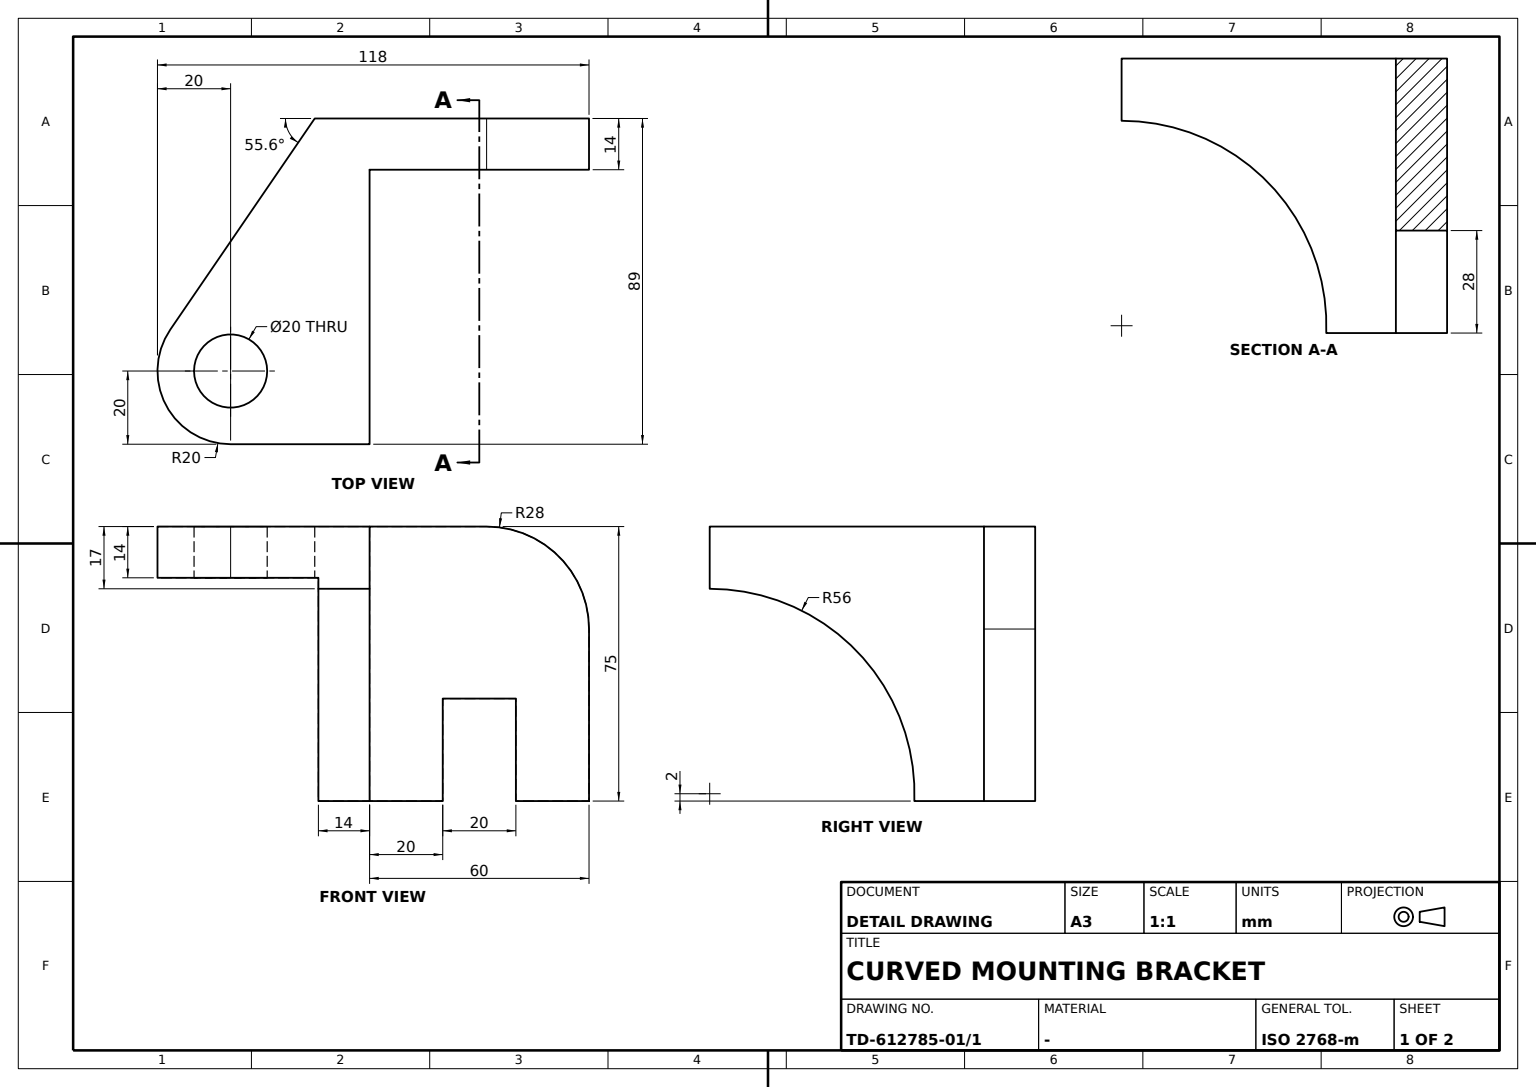
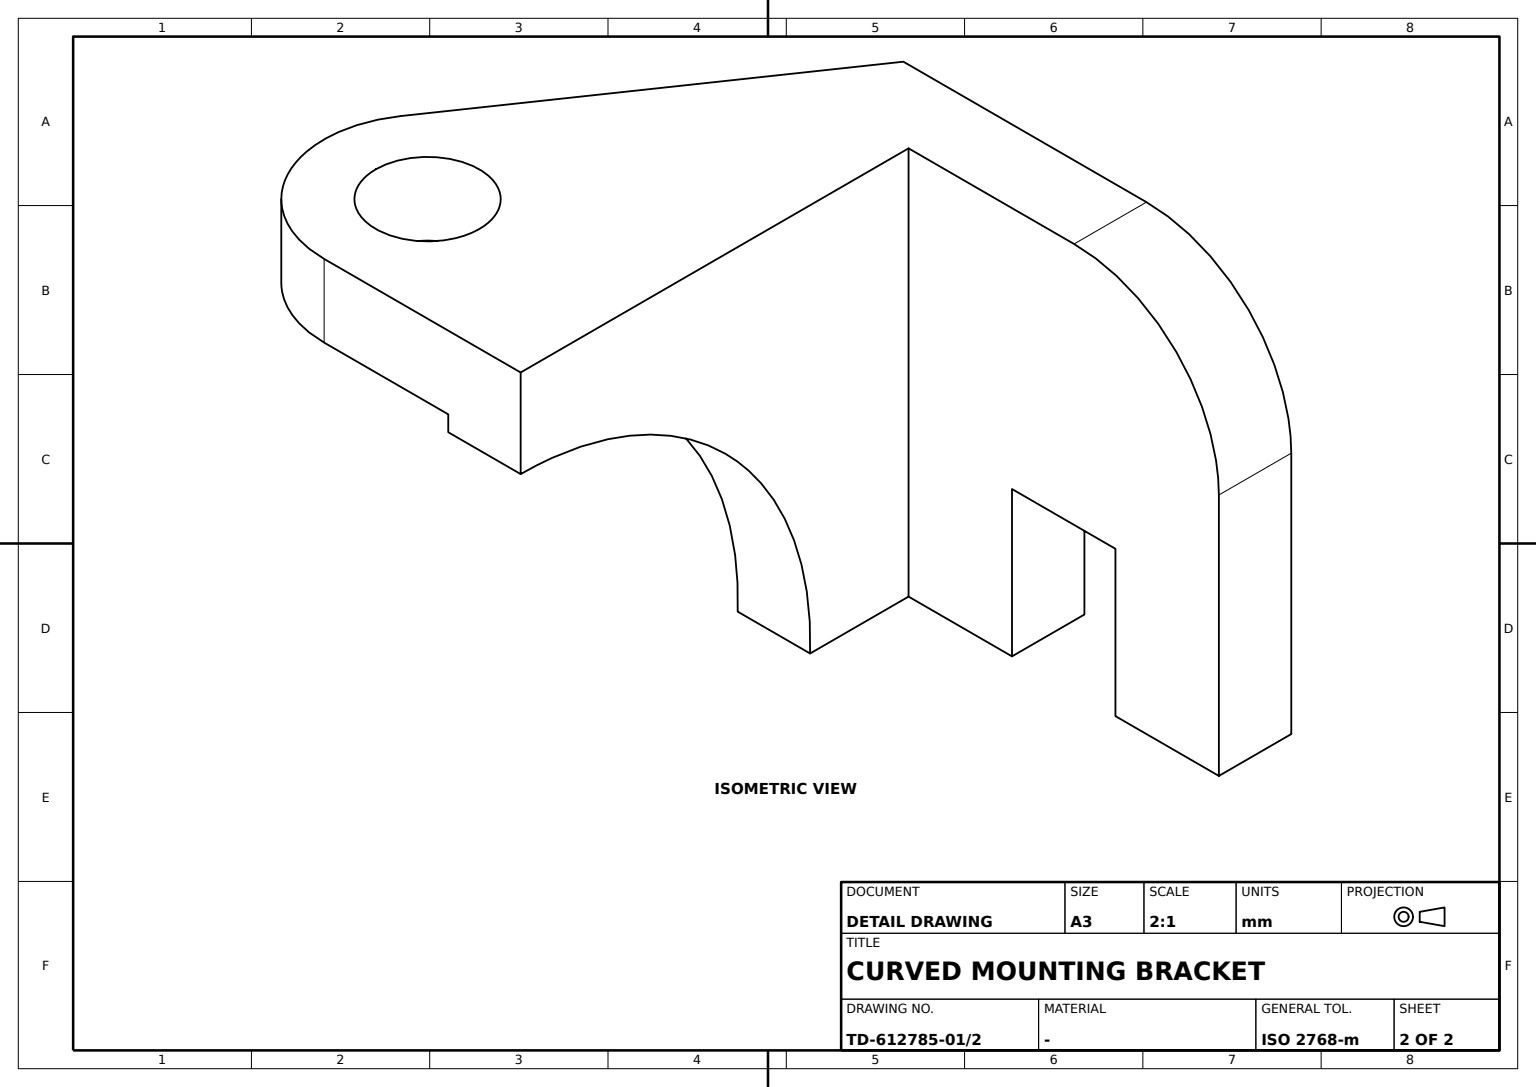
ISO-10303-21;
HEADER;
FILE_DESCRIPTION((''),'2;1');
FILE_NAME('','',(''),(''),'','','');
FILE_SCHEMA(('AUTOMOTIVE_DESIGN'));
ENDSEC;
DATA;
#1=APPLICATION_CONTEXT('');
#2=PRODUCT_CONTEXT('',#1,'mechanical');
#3=PRODUCT('','','',(#2));
#4=PRODUCT_DEFINITION_FORMATION('','',#3);
#5=PRODUCT_DEFINITION_CONTEXT('',#1,'design');
#6=PRODUCT_DEFINITION('','',#4,#5);
#7=PRODUCT_DEFINITION_SHAPE('','',#6);
#8=(LENGTH_UNIT()NAMED_UNIT(*)SI_UNIT(.MILLI.,.METRE.));
#9=(NAMED_UNIT(*)PLANE_ANGLE_UNIT()SI_UNIT($,.RADIAN.));
#10=(NAMED_UNIT(*)SI_UNIT($,.STERADIAN.)SOLID_ANGLE_UNIT());
#11=UNCERTAINTY_MEASURE_WITH_UNIT(LENGTH_MEASURE(0.005),#8,'distance_accuracy_value','');
#12=(GEOMETRIC_REPRESENTATION_CONTEXT(3)GLOBAL_UNCERTAINTY_ASSIGNED_CONTEXT((#11))GLOBAL_UNIT_ASSIGNED_CONTEXT((#8,#9,#10))REPRESENTATION_CONTEXT('',''));
#13=CARTESIAN_POINT('',(10.,0.,-37.5));
#14=VERTEX_POINT('',#13);
#15=CARTESIAN_POINT('',(10.,-14.,-37.5));
#16=VERTEX_POINT('',#15);
#17=CARTESIAN_POINT('',(10.,-29.,-37.5));
#18=DIRECTION('',(0.,1.,0.));
#19=VECTOR('',#18,1000.);
#20=LINE('',#17,#19);
#21=EDGE_CURVE('',#14,#16,#20,.F.);
#22=ORIENTED_EDGE('',*,*,#21,.T.);
#23=CARTESIAN_POINT('',(10.,-14.,-9.5));
#24=VERTEX_POINT('',#23);
#25=CARTESIAN_POINT('',(10.,-14.,0.));
#26=DIRECTION('',(0.,0.,-1.));
#27=VECTOR('',#26,1000.);
#28=LINE('',#25,#27);
#29=EDGE_CURVE('',#24,#16,#28,.T.);
#30=ORIENTED_EDGE('',*,*,#29,.F.);
#31=CARTESIAN_POINT('',(10.,0.,-9.5));
#32=VERTEX_POINT('',#31);
#33=CARTESIAN_POINT('',(10.,-29.,-9.5));
#34=LINE('',#33,#19);
#35=EDGE_CURVE('',#32,#24,#34,.F.);
#36=ORIENTED_EDGE('',*,*,#35,.F.);
#37=CARTESIAN_POINT('',(10.,0.,37.5));
#38=LINE('',#37,#27);
#39=EDGE_CURVE('',#32,#14,#38,.T.);
#40=ORIENTED_EDGE('',*,*,#39,.T.);
#41=EDGE_LOOP('',(#22,#30,#36,#40));
#42=FACE_BOUND('',#41,.T.);
#43=DIRECTION('',(1.,0.,0.));
#44=AXIS2_PLACEMENT_3D('',#33,#43,#26);
#45=PLANE('',#44);
#46=ADVANCED_FACE('',(#42),#45,.F.);
#47=CARTESIAN_POINT('',(-30.,-89.,20.5));
#48=VERTEX_POINT('',#47);
#49=CARTESIAN_POINT('',(-44.,-89.,20.5));
#50=VERTEX_POINT('',#49);
#51=DIRECTION('',(-1.,0.,0.));
#52=VECTOR('',#51,1000.);
#53=LINE('',#47,#52);
#54=EDGE_CURVE('',#48,#50,#53,.T.);
#55=ORIENTED_EDGE('',*,*,#54,.T.);
#56=CARTESIAN_POINT('',(-44.,-33.035726,-37.5));
#57=VERTEX_POINT('',#56);
#58=CARTESIAN_POINT('',(-44.,-89.,-35.5));
#59=DIRECTION('',(0.,0.,1.));
#60=AXIS2_PLACEMENT_3D('',#58,#51,#59);
#61=CIRCLE('',#60,56.);
#62=EDGE_CURVE('',#50,#57,#61,.T.);
#63=ORIENTED_EDGE('',*,*,#62,.T.);
#64=CARTESIAN_POINT('',(-30.,-33.035726,-37.5));
#65=VERTEX_POINT('',#64);
#66=CARTESIAN_POINT('',(-73.,-33.035726,-37.5));
#67=VECTOR('',#43,1000.);
#68=LINE('',#66,#67);
#69=EDGE_CURVE('',#57,#65,#68,.T.);
#70=ORIENTED_EDGE('',*,*,#69,.T.);
#71=CARTESIAN_POINT('',(-30.,-89.,-35.5));
#72=AXIS2_PLACEMENT_3D('',#71,#43,#18);
#73=CIRCLE('',#72,56.);
#74=EDGE_CURVE('',#65,#48,#73,.T.);
#75=ORIENTED_EDGE('',*,*,#74,.T.);
#76=EDGE_LOOP('',(#55,#63,#70,#75));
#77=FACE_BOUND('',#76,.T.);
#78=CARTESIAN_POINT('',(-73.,-89.,-35.5));
#79=AXIS2_PLACEMENT_3D('',#78,#43,#26);
#80=CYLINDRICAL_SURFACE('',#79,56.);
#81=ADVANCED_FACE('',(#77),#80,.F.);
#82=CARTESIAN_POINT('',(-68.,-89.,37.5));
#83=VERTEX_POINT('',#82);
#84=CARTESIAN_POINT('',(-84.503096,-57.701867,37.5));
#85=VERTEX_POINT('',#84);
#86=CARTESIAN_POINT('',(-68.,-69.,37.5));
#87=AXIS2_PLACEMENT_3D('',#86,#26,#43);
#88=CIRCLE('',#87,20.);
#89=EDGE_CURVE('',#83,#85,#88,.T.);
#90=ORIENTED_EDGE('',*,*,#89,.T.);
#91=CARTESIAN_POINT('',(-84.503096,-57.701867,23.5));
#92=VERTEX_POINT('',#91);
#93=LINE('',#84,#27);
#94=EDGE_CURVE('',#85,#92,#93,.T.);
#95=ORIENTED_EDGE('',*,*,#94,.T.);
#96=CARTESIAN_POINT('',(-68.,-89.,23.5));
#97=VERTEX_POINT('',#96);
#98=CARTESIAN_POINT('',(-68.,-69.,23.5));
#99=AXIS2_PLACEMENT_3D('',#98,#26,#43);
#100=CIRCLE('',#99,20.);
#101=EDGE_CURVE('',#97,#92,#100,.T.);
#102=ORIENTED_EDGE('',*,*,#101,.F.);
#103=LINE('',#82,#27);
#104=EDGE_CURVE('',#83,#97,#103,.T.);
#105=ORIENTED_EDGE('',*,*,#104,.F.);
#106=EDGE_LOOP('',(#90,#95,#102,#105));
#107=FACE_BOUND('',#106,.T.);
#108=AXIS2_PLACEMENT_3D('',#86,#26,#51);
#109=CYLINDRICAL_SURFACE('',#108,20.);
#110=ADVANCED_FACE('',(#107),#109,.T.);
#111=CARTESIAN_POINT('',(-30.,-89.,37.5));
#112=VERTEX_POINT('',#111);
#113=CARTESIAN_POINT('',(-44.,-89.,37.5));
#114=LINE('',#113,#67);
#115=EDGE_CURVE('',#112,#83,#114,.F.);
#116=ORIENTED_EDGE('',*,*,#115,.T.);
#117=ORIENTED_EDGE('',*,*,#104,.T.);
#118=CARTESIAN_POINT('',(-44.,-89.,23.5));
#119=VERTEX_POINT('',#118);
#120=CARTESIAN_POINT('',(-30.,-89.,23.5));
#121=LINE('',#120,#52);
#122=EDGE_CURVE('',#119,#97,#121,.T.);
#123=ORIENTED_EDGE('',*,*,#122,.F.);
#124=VECTOR('',#59,1000.);
#125=LINE('',#49,#124);
#126=EDGE_CURVE('',#50,#119,#125,.T.);
#127=ORIENTED_EDGE('',*,*,#126,.F.);
#128=ORIENTED_EDGE('',*,*,#54,.F.);
#129=LINE('',#111,#27);
#130=EDGE_CURVE('',#48,#112,#129,.F.);
#131=ORIENTED_EDGE('',*,*,#130,.T.);
#132=EDGE_LOOP('',(#116,#117,#123,#127,#128,#131));
#133=FACE_BOUND('',#132,.T.);
#134=CARTESIAN_POINT('',(0.,-89.,0.));
#135=AXIS2_PLACEMENT_3D('',#134,#18,#59);
#136=PLANE('',#135);
#137=ADVANCED_FACE('',(#133),#136,.F.);
#138=CARTESIAN_POINT('',(-78.,-69.,37.5));
#139=VERTEX_POINT('',#138);
#140=CIRCLE('',#108,10.);
#141=EDGE_CURVE('',#139,#139,#140,.T.);
#142=ORIENTED_EDGE('',*,*,#141,.T.);
#143=EDGE_LOOP('',(#142));
#144=FACE_BOUND('',#143,.T.);
#145=CARTESIAN_POINT('',(-30.,-14.,37.5));
#146=VERTEX_POINT('',#145);
#147=CARTESIAN_POINT('',(2.,-14.,37.5));
#148=VERTEX_POINT('',#147);
#149=LINE('',#145,#67);
#150=EDGE_CURVE('',#146,#148,#149,.T.);
#151=ORIENTED_EDGE('',*,*,#150,.T.);
#152=CARTESIAN_POINT('',(2.,0.,37.5));
#153=VERTEX_POINT('',#152);
#154=CARTESIAN_POINT('',(2.,-89.,37.5));
#155=LINE('',#154,#19);
#156=EDGE_CURVE('',#148,#153,#155,.T.);
#157=ORIENTED_EDGE('',*,*,#156,.T.);
#158=CARTESIAN_POINT('',(-45.,0.,37.5));
#159=VERTEX_POINT('',#158);
#160=LINE('',#158,#67);
#161=EDGE_CURVE('',#159,#153,#160,.T.);
#162=ORIENTED_EDGE('',*,*,#161,.F.);
#163=DIRECTION('',(0.564906674,0.825154804,0.));
#164=VECTOR('',#163,1000.);
#165=LINE('',#84,#164);
#166=EDGE_CURVE('',#85,#159,#165,.T.);
#167=ORIENTED_EDGE('',*,*,#166,.F.);
#168=ORIENTED_EDGE('',*,*,#89,.F.);
#169=ORIENTED_EDGE('',*,*,#115,.F.);
#170=LINE('',#111,#19);
#171=EDGE_CURVE('',#112,#146,#170,.T.);
#172=ORIENTED_EDGE('',*,*,#171,.T.);
#173=EDGE_LOOP('',(#151,#157,#162,#167,#168,#169,#172));
#174=FACE_BOUND('',#173,.T.);
#175=AXIS2_PLACEMENT_3D('',#113,#59,#43);
#176=PLANE('',#175);
#177=ADVANCED_FACE('',(#144,#174),#176,.T.);
#178=CARTESIAN_POINT('',(-78.,-69.,23.5));
#179=VERTEX_POINT('',#178);
#180=AXIS2_PLACEMENT_3D('',#98,#26,#51);
#181=CIRCLE('',#180,10.);
#182=EDGE_CURVE('',#179,#179,#181,.T.);
#183=ORIENTED_EDGE('',*,*,#182,.F.);
#184=EDGE_LOOP('',(#183));
#185=FACE_BOUND('',#184,.T.);
#186=CARTESIAN_POINT('',(-45.,0.,23.5));
#187=VERTEX_POINT('',#186);
#188=CARTESIAN_POINT('',(-44.,0.,23.5));
#189=VERTEX_POINT('',#188);
#190=LINE('',#186,#67);
#191=EDGE_CURVE('',#187,#189,#190,.T.);
#192=ORIENTED_EDGE('',*,*,#191,.T.);
#193=CARTESIAN_POINT('',(-44.,-69.,23.5));
#194=LINE('',#193,#19);
#195=EDGE_CURVE('',#119,#189,#194,.T.);
#196=ORIENTED_EDGE('',*,*,#195,.F.);
#197=ORIENTED_EDGE('',*,*,#122,.T.);
#198=ORIENTED_EDGE('',*,*,#101,.T.);
#199=LINE('',#91,#164);
#200=EDGE_CURVE('',#92,#187,#199,.T.);
#201=ORIENTED_EDGE('',*,*,#200,.T.);
#202=EDGE_LOOP('',(#192,#196,#197,#198,#201));
#203=FACE_BOUND('',#202,.T.);
#204=PLANE('',#180);
#205=ADVANCED_FACE('',(#185,#203),#204,.T.);
#206=CARTESIAN_POINT('',(-10.,-14.,-9.5));
#207=VERTEX_POINT('',#206);
#208=CARTESIAN_POINT('',(0.,-14.,-9.5));
#209=LINE('',#208,#67);
#210=EDGE_CURVE('',#207,#24,#209,.T.);
#211=ORIENTED_EDGE('',*,*,#210,.F.);
#212=CARTESIAN_POINT('',(-10.,0.,-9.5));
#213=VERTEX_POINT('',#212);
#214=CARTESIAN_POINT('',(-10.,-29.,-9.5));
#215=LINE('',#214,#19);
#216=EDGE_CURVE('',#213,#207,#215,.F.);
#217=ORIENTED_EDGE('',*,*,#216,.F.);
#218=CARTESIAN_POINT('',(-45.,0.,-9.5));
#219=LINE('',#218,#67);
#220=EDGE_CURVE('',#213,#32,#219,.T.);
#221=ORIENTED_EDGE('',*,*,#220,.T.);
#222=ORIENTED_EDGE('',*,*,#35,.T.);
#223=EDGE_LOOP('',(#211,#217,#221,#222));
#224=FACE_BOUND('',#223,.T.);
#225=AXIS2_PLACEMENT_3D('',#214,#59,#43);
#226=PLANE('',#225);
#227=ADVANCED_FACE('',(#224),#226,.F.);
#228=CARTESIAN_POINT('',(30.,-14.,-37.5));
#229=VERTEX_POINT('',#228);
#230=LINE('',#228,#52);
#231=EDGE_CURVE('',#229,#16,#230,.T.);
#232=ORIENTED_EDGE('',*,*,#231,.F.);
#233=CARTESIAN_POINT('',(30.,-14.,9.5));
#234=VERTEX_POINT('',#233);
#235=CARTESIAN_POINT('',(30.,-14.,37.5));
#236=LINE('',#235,#27);
#237=EDGE_CURVE('',#234,#229,#236,.T.);
#238=ORIENTED_EDGE('',*,*,#237,.F.);
#239=CARTESIAN_POINT('',(2.,-14.,9.5));
#240=AXIS2_PLACEMENT_3D('',#239,#18,#59);
#241=CIRCLE('',#240,28.);
#242=EDGE_CURVE('',#234,#148,#241,.F.);
#243=ORIENTED_EDGE('',*,*,#242,.T.);
#244=ORIENTED_EDGE('',*,*,#150,.F.);
#245=CARTESIAN_POINT('',(-30.,-14.,-37.5));
#246=VERTEX_POINT('',#245);
#247=LINE('',#145,#27);
#248=EDGE_CURVE('',#246,#146,#247,.F.);
#249=ORIENTED_EDGE('',*,*,#248,.F.);
#250=CARTESIAN_POINT('',(-10.,-14.,-37.5));
#251=VERTEX_POINT('',#250);
#252=EDGE_CURVE('',#251,#246,#230,.T.);
#253=ORIENTED_EDGE('',*,*,#252,.F.);
#254=CARTESIAN_POINT('',(-10.,-14.,0.));
#255=LINE('',#254,#124);
#256=EDGE_CURVE('',#251,#207,#255,.T.);
#257=ORIENTED_EDGE('',*,*,#256,.T.);
#258=ORIENTED_EDGE('',*,*,#210,.T.);
#259=ORIENTED_EDGE('',*,*,#29,.T.);
#260=EDGE_LOOP('',(#232,#238,#243,#244,#249,#253,#257,#258,#259));
#261=FACE_BOUND('',#260,.T.);
#262=CARTESIAN_POINT('',(0.,-14.,0.));
#263=AXIS2_PLACEMENT_3D('',#262,#18,#59);
#264=PLANE('',#263);
#265=ADVANCED_FACE('',(#261),#264,.F.);
#266=ORIENTED_EDGE('',*,*,#182,.T.);
#267=EDGE_LOOP('',(#266));
#268=FACE_BOUND('',#267,.T.);
#269=ORIENTED_EDGE('',*,*,#141,.F.);
#270=EDGE_LOOP('',(#269));
#271=FACE_BOUND('',#270,.T.);
#272=CYLINDRICAL_SURFACE('',#108,10.);
#273=ADVANCED_FACE('',(#268,#271),#272,.F.);
#274=ORIENTED_EDGE('',*,*,#248,.T.);
#275=ORIENTED_EDGE('',*,*,#171,.F.);
#276=ORIENTED_EDGE('',*,*,#130,.F.);
#277=ORIENTED_EDGE('',*,*,#74,.F.);
#278=CARTESIAN_POINT('',(-30.,0.,-37.5));
#279=DIRECTION('',(0.,-1.,0.));
#280=VECTOR('',#279,1000.);
#281=LINE('',#278,#280);
#282=EDGE_CURVE('',#246,#65,#281,.T.);
#283=ORIENTED_EDGE('',*,*,#282,.F.);
#284=EDGE_LOOP('',(#274,#275,#276,#277,#283));
#285=FACE_BOUND('',#284,.T.);
#286=AXIS2_PLACEMENT_3D('',#111,#43,#26);
#287=PLANE('',#286);
#288=ADVANCED_FACE('',(#285),#287,.T.);
#289=ORIENTED_EDGE('',*,*,#94,.F.);
#290=ORIENTED_EDGE('',*,*,#166,.T.);
#291=LINE('',#158,#27);
#292=EDGE_CURVE('',#159,#187,#291,.T.);
#293=ORIENTED_EDGE('',*,*,#292,.T.);
#294=ORIENTED_EDGE('',*,*,#200,.F.);
#295=EDGE_LOOP('',(#289,#290,#293,#294));
#296=FACE_BOUND('',#295,.T.);
#297=DIRECTION('',(-0.825154804,0.564906674,0.));
#298=DIRECTION('',(-0.564906674,-0.825154804,0.));
#299=AXIS2_PLACEMENT_3D('',#84,#297,#298);
#300=PLANE('',#299);
#301=ADVANCED_FACE('',(#296),#300,.T.);
#302=CARTESIAN_POINT('',(30.,0.,-37.5));
#303=VERTEX_POINT('',#302);
#304=LINE('',#278,#52);
#305=EDGE_CURVE('',#303,#14,#304,.T.);
#306=ORIENTED_EDGE('',*,*,#305,.F.);
#307=LINE('',#228,#19);
#308=EDGE_CURVE('',#229,#303,#307,.T.);
#309=ORIENTED_EDGE('',*,*,#308,.F.);
#310=ORIENTED_EDGE('',*,*,#231,.T.);
#311=ORIENTED_EDGE('',*,*,#21,.F.);
#312=EDGE_LOOP('',(#306,#309,#310,#311));
#313=FACE_BOUND('',#312,.T.);
#314=AXIS2_PLACEMENT_3D('',#278,#26,#18);
#315=PLANE('',#314);
#316=ADVANCED_FACE('',(#313),#315,.T.);
#317=ORIENTED_EDGE('',*,*,#252,.T.);
#318=ORIENTED_EDGE('',*,*,#282,.T.);
#319=ORIENTED_EDGE('',*,*,#69,.F.);
#320=CARTESIAN_POINT('',(-44.,0.,-37.5));
#321=VERTEX_POINT('',#320);
#322=LINE('',#320,#280);
#323=EDGE_CURVE('',#321,#57,#322,.T.);
#324=ORIENTED_EDGE('',*,*,#323,.F.);
#325=CARTESIAN_POINT('',(-10.,0.,-37.5));
#326=VERTEX_POINT('',#325);
#327=EDGE_CURVE('',#326,#321,#304,.T.);
#328=ORIENTED_EDGE('',*,*,#327,.F.);
#329=CARTESIAN_POINT('',(-10.,-29.,-37.5));
#330=LINE('',#329,#19);
#331=EDGE_CURVE('',#326,#251,#330,.F.);
#332=ORIENTED_EDGE('',*,*,#331,.T.);
#333=EDGE_LOOP('',(#317,#318,#319,#324,#328,#332));
#334=FACE_BOUND('',#333,.T.);
#335=ADVANCED_FACE('',(#334),#315,.T.);
#336=ORIENTED_EDGE('',*,*,#62,.F.);
#337=ORIENTED_EDGE('',*,*,#126,.T.);
#338=ORIENTED_EDGE('',*,*,#195,.T.);
#339=CARTESIAN_POINT('',(-44.,0.,37.5));
#340=LINE('',#339,#27);
#341=EDGE_CURVE('',#189,#321,#340,.T.);
#342=ORIENTED_EDGE('',*,*,#341,.T.);
#343=ORIENTED_EDGE('',*,*,#323,.T.);
#344=EDGE_LOOP('',(#336,#337,#338,#342,#343));
#345=FACE_BOUND('',#344,.T.);
#346=AXIS2_PLACEMENT_3D('',#49,#51,#59);
#347=PLANE('',#346);
#348=ADVANCED_FACE('',(#345),#347,.T.);
#349=ORIENTED_EDGE('',*,*,#256,.F.);
#350=ORIENTED_EDGE('',*,*,#331,.F.);
#351=CARTESIAN_POINT('',(-10.,0.,37.5));
#352=LINE('',#351,#124);
#353=EDGE_CURVE('',#326,#213,#352,.T.);
#354=ORIENTED_EDGE('',*,*,#353,.T.);
#355=ORIENTED_EDGE('',*,*,#216,.T.);
#356=EDGE_LOOP('',(#349,#350,#354,#355));
#357=FACE_BOUND('',#356,.T.);
#358=AXIS2_PLACEMENT_3D('',#329,#51,#59);
#359=PLANE('',#358);
#360=ADVANCED_FACE('',(#357),#359,.F.);
#361=CARTESIAN_POINT('',(30.,0.,9.5));
#362=VERTEX_POINT('',#361);
#363=CARTESIAN_POINT('',(2.,0.,9.5));
#364=AXIS2_PLACEMENT_3D('',#363,#18,#59);
#365=CIRCLE('',#364,28.);
#366=EDGE_CURVE('',#153,#362,#365,.T.);
#367=ORIENTED_EDGE('',*,*,#366,.F.);
#368=ORIENTED_EDGE('',*,*,#156,.F.);
#369=ORIENTED_EDGE('',*,*,#242,.F.);
#370=LINE('',#233,#19);
#371=EDGE_CURVE('',#362,#234,#370,.F.);
#372=ORIENTED_EDGE('',*,*,#371,.F.);
#373=EDGE_LOOP('',(#367,#368,#369,#372));
#374=FACE_BOUND('',#373,.T.);
#375=CARTESIAN_POINT('',(2.,-89.,9.5));
#376=AXIS2_PLACEMENT_3D('',#375,#18,#59);
#377=CYLINDRICAL_SURFACE('',#376,28.);
#378=ADVANCED_FACE('',(#374),#377,.T.);
#379=ORIENTED_EDGE('',*,*,#39,.F.);
#380=ORIENTED_EDGE('',*,*,#220,.F.);
#381=ORIENTED_EDGE('',*,*,#353,.F.);
#382=ORIENTED_EDGE('',*,*,#327,.T.);
#383=ORIENTED_EDGE('',*,*,#341,.F.);
#384=ORIENTED_EDGE('',*,*,#191,.F.);
#385=ORIENTED_EDGE('',*,*,#292,.F.);
#386=ORIENTED_EDGE('',*,*,#161,.T.);
#387=ORIENTED_EDGE('',*,*,#366,.T.);
#388=CARTESIAN_POINT('',(30.,0.,37.5));
#389=LINE('',#388,#27);
#390=EDGE_CURVE('',#362,#303,#389,.T.);
#391=ORIENTED_EDGE('',*,*,#390,.T.);
#392=ORIENTED_EDGE('',*,*,#305,.T.);
#393=EDGE_LOOP('',(#379,#380,#381,#382,#383,#384,#385,#386,#387,#391,#392));
#394=FACE_BOUND('',#393,.T.);
#395=AXIS2_PLACEMENT_3D('',#158,#18,#59);
#396=PLANE('',#395);
#397=ADVANCED_FACE('',(#394),#396,.T.);
#398=ORIENTED_EDGE('',*,*,#371,.T.);
#399=ORIENTED_EDGE('',*,*,#237,.T.);
#400=ORIENTED_EDGE('',*,*,#308,.T.);
#401=ORIENTED_EDGE('',*,*,#390,.F.);
#402=EDGE_LOOP('',(#398,#399,#400,#401));
#403=FACE_BOUND('',#402,.T.);
#404=AXIS2_PLACEMENT_3D('',#235,#43,#26);
#405=PLANE('',#404);
#406=ADVANCED_FACE('',(#403),#405,.T.);
#407=CLOSED_SHELL('',(#46,#81,#110,#137,#177,#205,#227,#265,#273,#288,#301,#316,#335,#348,#360,#378,#397,#406));
#408=MANIFOLD_SOLID_BREP('',#407);
#409=ADVANCED_BREP_SHAPE_REPRESENTATION('',(#408),#12);
#410=SHAPE_DEFINITION_REPRESENTATION(#7,#409);
ENDSEC;
END-ISO-10303-21;
